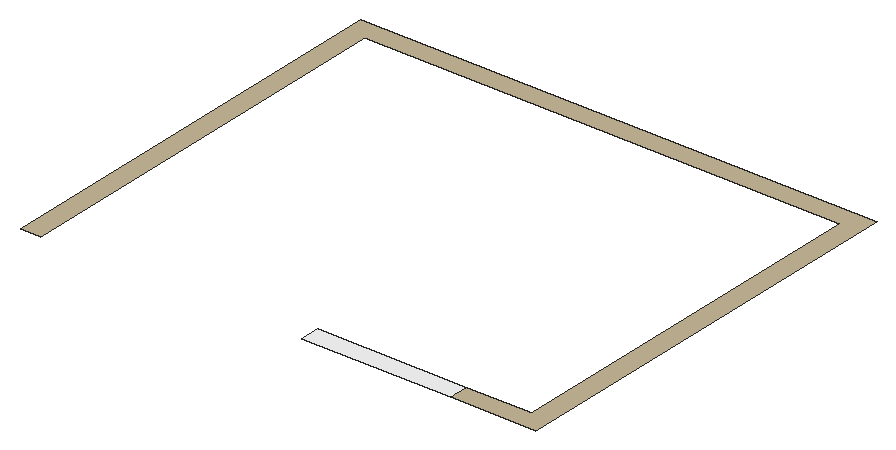
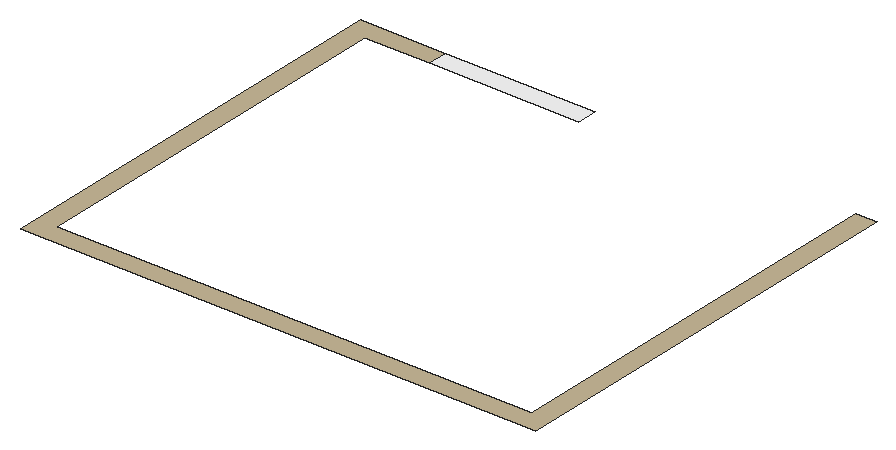
# SketchUp Ruby script. Lengths in inches.
U = 1.inch
M = Sketchup.active_model
def pt(a) = Geom::Point3d.new(a.map { |v| v * U })
def face(e, loops, mat)
  f = e.add_face(loops[0].map { |a| pt(a) })
  loops[1..].each { |l| e.add_face(l.map { |a| pt(a) }).erase! }
  f.material = f.back_material = mat if mat
  f
end
# faces: each face lists its corners as indices into pts; further lists are holes
def faces(e, pts, list, mat = nil) = list.each { |f| face(e, (f[0].is_a?(Array) ? f : [f]).map { |l| l.map { |i| pts[i] } }, mat) }
# xy, xz, yz: faces in a plane at the given z, y or x. An outline is a flat list of corners, or four numbers for a rectangle; further outlines are holes
def ring(l) = l.size == 4 ? [[l[0], l[1]], [l[2], l[1]], [l[2], l[3]], [l[0], l[3]]] : l.each_slice(2).to_a
def flat(e, list, mat, &to3) = list.each { |f| face(e, (f[0].is_a?(Array) ? f : [f]).map { |l| ring(l).map { |u, v| to3.(u, v) } }, mat) }
def xy(e, z, list, mat = nil) = flat(e, list, mat) { |x, y| [x, y, z] }
def xz(e, y, list, mat = nil) = flat(e, list, mat) { |x, z| [x, y, z] }
def yz(e, x, list, mat = nil) = flat(e, list, mat) { |y, z| [x, y, z] }
def lines(e, pts, list) = list.each { |a, b| e.add_line(pt(pts[a]), pt(pts[b])) }
# prism: a flat outline (further loops are holes) pulled along v
def prism(e, loops, v, mat = nil)
  f = face(e, loops, mat); d = Geom::Vector3d.new(v.map { |x| x * U })
  f.pushpull(f.normal.samedirection?(d) ? d.length : -d.length)
end
def box(e, o, s, mat = nil) = prism(e, [[o, [o[0] + s[0], o[1], o[2]], [o[0] + s[0], o[1] + s[1], o[2]], [o[0], o[1] + s[1], o[2]]]], [0, 0, s[2]], mat)
def at(x, y, z, deg = 0) = Geom::Transformation.translation(pt([x, y, z])) * Geom::Transformation.rotation(ORIGIN, Z_AXIS, deg.degrees)
def axes(o, x, y, z) = Geom::Transformation.new([*x, 0, *y, 0, *z, 0, *pt(o).to_a, 1])
def part(name) = M.definitions.add(name)
# library, detail: a bought-in or finely detailed component or shape, given as its bounding box
def library(name, o, s) = part(name).tap { |d| box(d.entities, o, s) }
def detail(e, o, s) = box(e.add_group.entities, o, s)
def put(e, d, t, mat = nil) = e.add_instance(d, t).tap { |i| i.material = mat if mat }
def group(e, t, mat = nil) = e.add_group.tap { |g| g.transformation = t; g.material = mat if mat }.entities
root = M.entities
M.materials.add("[Blinds Vertical Stripe Gray]1").color = [252, 252, 252]
M.materials.add("[Quartz Light Brown]").color = [199, 184, 152]
xy(root,57.8125,[[206.19,96.24,315.3,111]],"[Blinds Vertical Stripe Gray]1")
xy(root,57.8125,[[0,96.24,14.76,96.24,14.76,393.42,363.05,393.42,363.05,111,315.3,111,315.3,96.24,377.8125,96.24,377.8125,408.18,0,408.18]],"[Quartz Light Brown]")
